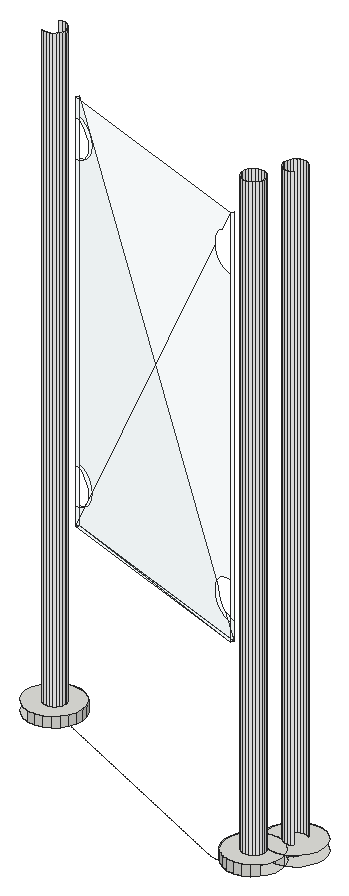
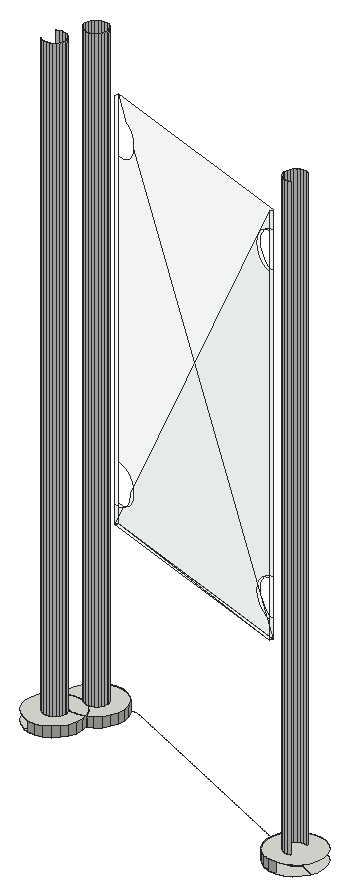
# SketchUp Ruby script. Lengths in inches.
U = 1.inch
M = Sketchup.active_model
def pt(a) = Geom::Point3d.new(a.map { |v| v * U })
def face(e, loops, mat)
  f = e.add_face(loops[0].map { |a| pt(a) })
  loops[1..].each { |l| e.add_face(l.map { |a| pt(a) }).erase! }
  f.material = f.back_material = mat if mat
  f
end
# faces: each face lists its corners as indices into pts; further lists are holes
def faces(e, pts, list, mat = nil) = list.each { |f| face(e, (f[0].is_a?(Array) ? f : [f]).map { |l| l.map { |i| pts[i] } }, mat) }
# xy, xz, yz: faces in a plane at the given z, y or x. An outline is a flat list of corners, or four numbers for a rectangle; further outlines are holes
def ring(l) = l.size == 4 ? [[l[0], l[1]], [l[2], l[1]], [l[2], l[3]], [l[0], l[3]]] : l.each_slice(2).to_a
def flat(e, list, mat, &to3) = list.each { |f| face(e, (f[0].is_a?(Array) ? f : [f]).map { |l| ring(l).map { |u, v| to3.(u, v) } }, mat) }
def xy(e, z, list, mat = nil) = flat(e, list, mat) { |x, y| [x, y, z] }
def xz(e, y, list, mat = nil) = flat(e, list, mat) { |x, z| [x, y, z] }
def yz(e, x, list, mat = nil) = flat(e, list, mat) { |y, z| [x, y, z] }
def lines(e, pts, list) = list.each { |a, b| e.add_line(pt(pts[a]), pt(pts[b])) }
# prism: a flat outline (further loops are holes) pulled along v
def prism(e, loops, v, mat = nil)
  f = face(e, loops, mat); d = Geom::Vector3d.new(v.map { |x| x * U })
  f.pushpull(f.normal.samedirection?(d) ? d.length : -d.length)
end
def box(e, o, s, mat = nil) = prism(e, [[o, [o[0] + s[0], o[1], o[2]], [o[0] + s[0], o[1] + s[1], o[2]], [o[0], o[1] + s[1], o[2]]]], [0, 0, s[2]], mat)
def at(x, y, z, deg = 0) = Geom::Transformation.translation(pt([x, y, z])) * Geom::Transformation.rotation(ORIGIN, Z_AXIS, deg.degrees)
def axes(o, x, y, z) = Geom::Transformation.new([*x, 0, *y, 0, *z, 0, *pt(o).to_a, 1])
def part(name) = M.definitions.add(name)
# library, detail: a bought-in or finely detailed component or shape, given as its bounding box
def library(name, o, s) = part(name).tap { |d| box(d.entities, o, s) }
def detail(e, o, s) = box(e.add_group.entities, o, s)
def put(e, d, t, mat = nil) = e.add_instance(d, t).tap { |i| i.material = mat if mat }
def group(e, t, mat = nil) = e.add_group.tap { |g| g.transformation = t; g.material = mat if mat }.entities
root = M.entities
M.materials.add("Glass_Safety_01").color = [204, 235, 244]
M.materials["Glass_Safety_01"].alpha = 0.1
M.materials.add("[Color_000]").color = [255, 255, 255]
xy(root,321.267,[[[843.197,534.256,843.6,534.339,843.967,534.523,844.275,534.796,844.501,535.139,844.631,535.529,844.655,535.94,844.587,536.273,844.573,536.342,844.388,536.71,844.116,537.017,843.971,537.113,843.9,537.117,843.769,537.16,843.744,537.169,843.607,537.259,843.557,537.315,843.382,537.373,842.972,537.398,842.569,537.315,842.517,537.289,842.202,537.131,841.894,536.858,841.668,536.515,841.538,536.125,841.514,535.714,841.596,535.312,841.78,534.944,841.918,534.79,842.053,534.637,842.397,534.41,842.787,534.281],[843.13,535.199,842.965,535.208,842.846,535.248,842.901,535.313,842.956,535.387,843.006,535.464,843.051,535.544,843.221,535.902,843.393,536.298,843.547,536.247,843.606,536.18,843.68,536.033,843.713,535.872,843.703,535.708,843.651,535.552,843.561,535.415,843.4375,535.305,843.291,535.232],[843.393,536.298,843.332,536.319,843.133,536.45,843.204,536.446,843.36,536.394,843.418,536.355]],[841.918,534.79,841.962,534.793,842.053,534.807,842.143,534.826,842.231,534.851,842.318,534.882,842.402,534.918,842.484,534.96,842.5625,535.007,842.638,535.059,842.71,535.116,842.778,535.177,842.842,535.243,842.846,535.248,842.809,535.26,842.672,535.351,842.563,535.474,842.489,535.621,842.456,535.782,842.466,535.946,842.518,536.102,842.608,536.239,842.731,536.349,842.878,536.422,843.039,536.455,843.133,536.45,843.204,536.446,843.36,536.394,843.418,536.355,843.769,537.16,843.744,537.169,843.607,537.259,843.557,537.315,843.498,537.382,843.424,537.529,843.391,537.69,843.401,537.854,843.453,538.01,843.543,538.148,843.666,538.257,843.813,538.331,843.974,538.364,844.139,538.354,844.27,538.31,844.645,539.173,844.317,539.282,843.907,539.306,843.504,539.223,843.137,539.039,842.829,538.766,842.603,538.423,842.473,538.033,842.449,537.623,842.517,537.289,842.202,537.131,841.894,536.858,841.668,536.515,841.538,536.125,841.514,535.714,841.596,535.312,841.78,534.944],[842.846,535.248,842.901,535.313,842.956,535.387,843.006,535.464,843.051,535.544,843.221,535.902,843.393,536.298,843.332,536.319,843.133,536.45,843.039,536.455,842.878,536.422,842.731,536.349,842.608,536.239,842.518,536.102,842.466,535.946,842.456,535.782,842.489,535.621,842.563,535.474,842.672,535.351,842.809,535.26],[[844.132,536.165,843.722,536.189,843.547,536.247,843.497,536.303,843.418,536.355,843.36,536.394,843.204,536.446,843.133,536.45,842.988,536.545,842.715,536.852,842.531,537.22,842.517,537.289,842.449,537.623,842.473,538.033,842.603,538.423,842.829,538.766,843.137,539.039,843.504,539.223,843.907,539.306,844.317,539.282,844.645,539.173,844.707,539.152,845.051,538.926,845.323,538.618,845.508,538.251,845.59,537.848,845.566,537.4375,845.436,537.047,845.21,536.704,844.902,536.431,844.587,536.273,844.535,536.247],[844.064,537.107,844.226,537.14,844.373,537.214,844.496,537.323,844.586,537.46,844.638,537.616,844.648,537.78,844.615,537.941,844.541,538.088,844.432,538.211,844.295,538.302,844.27,538.31,843.798,537.227,843.971,537.113],[843.769,537.16,843.798,537.227,843.772,537.244,843.557,537.315,843.607,537.259,843.744,537.169]],[843.769,537.16,843.744,537.169,843.607,537.259,843.557,537.315,843.772,537.244,843.798,537.227],
  [843.798,537.227,844.27,538.31,844.139,538.354,843.974,538.364,843.813,538.331,843.666,538.257,843.543,538.148,843.453,538.01,843.401,537.854,843.391,537.69,843.424,537.529,843.498,537.382,843.557,537.315,843.772,537.244],[[827.381,539.408,827.783,539.491,828.151,539.675,828.458,539.948,828.685,540.291,828.705,540.352,828.815,540.681,828.839,541.092,828.756,541.494,828.572,541.862,828.299,542.169,827.956,542.396,827.566,542.525,827.156,542.55,826.753,542.467,826.385,542.283,826.078,542.01,825.851,541.667,825.83,541.603,825.722,541.277,825.697,540.866,825.78,540.464,825.964,540.096,826.237,539.789,826.58,539.5625,826.97,539.433],[827.313,540.351,827.149,540.36,826.993,540.412,826.856,540.503,826.747,540.626,826.673,540.773,826.64,540.934,826.65,541.098,826.693,541.228,826.701,541.254,826.792,541.391,826.915,541.501,827.062,541.574,827.223,541.607,827.387,541.598,827.543,541.546,827.681,541.455,827.79,541.332,827.863,541.185,827.896,541.024,827.887,540.86,827.843,540.727,827.835,540.704,827.744,540.567,827.621,540.457,827.474,540.384]],[828.705,540.352,828.815,540.681,828.839,541.092,828.756,541.494,828.572,541.862,828.299,542.169,827.956,542.396,827.566,542.525,827.156,542.55,826.753,542.467,826.385,542.283,826.078,542.01,825.851,541.667,825.83,541.603,826.693,541.228,826.701,541.254,826.792,541.391,826.915,541.501,827.062,541.574,827.223,541.607,827.387,541.598,827.543,541.546,827.681,541.455,827.79,541.332,827.863,541.185,827.896,541.024,827.887,540.86,827.843,540.727],[827.843,540.727,827.887,540.86,827.896,541.024,827.863,541.185,827.79,541.332,827.681,541.455,827.543,541.546,827.387,541.598,827.223,541.607,827.062,541.574,826.915,541.501,826.792,541.391,826.701,541.254,826.693,541.228]])
xy(root,321.267,[[843.13,535.199,842.965,535.208,842.846,535.248,842.901,535.313,842.956,535.387,843.006,535.464,843.051,535.544,843.221,535.902,843.393,536.298,843.547,536.247,843.606,536.18,843.68,536.033,843.713,535.872,843.703,535.708,843.651,535.552,843.561,535.415,843.4375,535.305,843.291,535.232],[843.547,536.247,843.393,536.298,843.418,536.355,843.497,536.303],[843.393,536.298,843.332,536.319,843.133,536.45,843.204,536.446,843.36,536.394,843.418,536.355],[844.064,537.107,843.971,537.113,843.798,537.227,844.27,538.31,844.295,538.302,844.432,538.211,844.541,538.088,844.615,537.941,844.648,537.78,844.638,537.616,844.586,537.46,844.496,537.323,844.373,537.214,844.226,537.14],[843.971,537.113,843.798,537.227,843.769,537.16,843.9,537.117],
  [827.313,540.351,827.474,540.384,827.621,540.457,827.744,540.567,827.835,540.704,827.843,540.727,826.693,541.228,826.65,541.098,826.64,540.934,826.673,540.773,826.747,540.626,826.856,540.503,826.993,540.412,827.149,540.36]],"[Color_000]")
xy(root,321.858,[[843.197,534.256,843.6,534.339,843.967,534.523,844.275,534.796,844.501,535.139,844.631,535.529,844.655,535.94,844.587,536.273,844.535,536.247,844.132,536.165,843.722,536.189,843.332,536.319,842.988,536.545,842.715,536.852,842.531,537.22,842.517,537.289,842.202,537.131,841.894,536.858,841.668,536.515,841.538,536.125,841.514,535.714,841.596,535.312,841.78,534.944,842.053,534.637,842.397,534.41,842.787,534.281],[844.132,536.165,844.535,536.247,844.587,536.273,844.573,536.342,844.388,536.71,844.116,537.017,843.772,537.244,843.382,537.373,842.972,537.398,842.569,537.315,842.517,537.289,842.531,537.22,842.715,536.852,842.988,536.545,843.332,536.319,843.722,536.189],[844.587,536.273,844.902,536.431,845.21,536.704,845.436,537.047,845.566,537.4375,845.59,537.848,845.508,538.251,845.323,538.618,845.051,538.926,844.707,539.152,844.317,539.282,843.907,539.306,843.504,539.223,843.137,539.039,842.829,538.766,842.603,538.423,842.473,538.033,842.449,537.623,842.517,537.289,842.569,537.315,842.972,537.398,843.382,537.373,843.772,537.244,844.116,537.017,844.388,536.71,844.573,536.342],[827.381,539.408,827.783,539.491,828.151,539.675,828.458,539.948,828.685,540.291,828.815,540.681,828.839,541.092,828.756,541.494,828.572,541.862,828.299,542.169,827.956,542.396,827.566,542.525,827.156,542.55,826.753,542.467,826.385,542.283,826.078,542.01,825.851,541.667,825.722,541.277,825.697,540.866,825.78,540.464,825.964,540.096,826.237,539.789,826.58,539.5625,826.97,539.433]])
xy(root,331.897,[[841.404,536.271,829.109,540.276,829.17,540.463],[841.404,536.271,829.17,540.463,841.465,536.458],[844.039,537.551,843.862,537.638,844.044,537.562],[844.044,537.562,843.862,537.638,843.867,537.648]],"Glass_Safety_01")
p = [[842.397,534.41,321.267],[842.787,534.281,321.267],[842.787,534.281,321.858],[842.397,534.41,321.858],[843.197,534.256,321.267],[843.197,534.256,321.858],
  [843.6,534.339,321.267],[843.6,534.339,321.858],[843.967,534.523,321.267],[843.967,534.523,321.858],[842.053,534.637,321.267],[842.053,534.637,321.858],
  [844.275,534.796,321.267],[844.275,534.796,321.858],[841.78,534.944,321.267],[841.918,534.79,321.267],[841.78,534.944,321.858],[841.596,535.312,321.267],
  [841.596,535.312,321.858],[842.809,535.26,321.267],[842.846,535.248,321.267],[842.965,535.208,321.267],[842.965,535.208,357.267],[842.809,535.26,357.267],
  [843.13,535.199,321.267],[843.13,535.199,357.267],[843.291,535.232,321.267],[843.291,535.232,357.267],[843.4375,535.305,321.267],[843.4375,535.305,357.267],
  [841.514,535.714,321.267],[841.514,535.714,321.858],[842.672,535.351,321.267],[842.672,535.351,357.267],[843.561,535.415,321.267],[843.561,535.415,357.267],
  [842.563,535.474,321.267],[842.563,535.474,357.267],[843.651,535.552,321.267],[843.651,535.552,357.267],[842.489,535.621,321.267],[842.489,535.621,357.267],
  [842.456,535.782,321.267],[842.456,535.782,357.267],[843.703,535.708,321.267],[843.703,535.708,357.267],[841.538,536.125,321.267],[841.538,536.125,321.858],
  [843.713,535.872,321.267],[843.713,535.872,357.267],[842.466,535.946,321.267],[842.466,535.946,357.267],[842.518,536.102,321.267],[842.518,536.102,357.267],
  [843.68,536.033,321.267],[843.68,536.033,357.267],[843.606,536.18,321.267],[843.606,536.18,357.267],[841.668,536.515,321.267],[841.668,536.515,321.858],
  [842.608,536.239,321.267],[842.608,536.239,357.267],[842.731,536.349,321.267],[842.731,536.349,357.267],[843.332,536.319,321.267],[843.393,536.298,321.267],
  [843.547,536.247,321.267],[843.722,536.189,321.267],[843.722,536.189,321.858],[843.332,536.319,321.858],[843.497,536.303,321.267],[843.497,536.303,357.267],
  [844.132,536.165,321.267],[844.132,536.165,321.858],[844.535,536.247,321.267],[844.535,536.247,321.858],[842.878,536.422,321.267],[842.878,536.422,357.267],
  [842.988,536.545,321.267],[843.133,536.45,321.267],[842.988,536.545,321.858],[843.418,536.355,321.267],[843.36,536.394,321.267],[843.36,536.394,357.267],
  [843.039,536.455,321.267],[843.039,536.455,357.267],[843.204,536.446,321.267],[843.204,536.446,357.267],[841.894,536.858,321.267],[841.894,536.858,321.858],
  [842.715,536.852,321.267],[842.715,536.852,321.858],[844.388,536.71,321.267],[844.116,537.017,321.267],[844.116,537.017,321.858],[844.388,536.71,321.858],
  [842.202,537.131,321.267],[842.202,537.131,321.858],[842.531,537.22,321.267],[842.531,537.22,321.858],[843.971,537.113,321.267],[843.798,537.227,321.267],
  [843.772,537.244,321.267],[843.772,537.244,321.858],[842.569,537.315,321.267],[842.517,537.289,321.267],[842.517,537.289,321.858],[842.569,537.315,321.858],
  [843.744,537.169,321.267],[843.769,537.16,321.267],[843.9,537.117,321.267],[843.9,537.117,357.267],[843.744,537.169,357.267],[844.064,537.107,321.267],
  [844.064,537.107,357.267],[844.226,537.14,321.267],[844.226,537.14,357.267],[844.373,537.214,321.267],[844.373,537.214,357.267],[842.449,537.623,321.267],
  [842.449,537.623,321.858],[843.557,537.315,321.267],[843.382,537.373,321.267],[843.382,537.373,321.858],[843.607,537.259,321.267],[843.607,537.259,357.267],
  [842.972,537.398,321.267],[842.972,537.398,321.858],[843.498,537.382,321.267],[843.498,537.382,357.267],[843.424,537.529,321.267],[843.424,537.529,357.267],
  [843.391,537.69,321.267],[843.391,537.69,357.267],[842.473,538.033,321.267],[842.473,538.033,321.858],[843.401,537.854,321.267],[843.401,537.854,357.267],
  [843.453,538.01,321.267],[843.453,538.01,357.267],[842.603,538.423,321.267],[842.603,538.423,321.858],[843.543,538.148,321.267],[843.543,538.148,357.267],
  [843.666,538.257,321.267],[843.666,538.257,357.267],[844.432,538.211,321.267],[844.295,538.302,321.267],[844.295,538.302,357.267],[844.432,538.211,357.267],
  [843.813,538.331,321.267],[843.813,538.331,357.267],[843.974,538.364,321.267],[843.974,538.364,357.267],[844.27,538.31,321.267],[844.139,538.354,321.267],
  [844.139,538.354,357.267],[842.829,538.766,321.267],[842.829,538.766,321.858],[843.137,539.039,321.267],[843.137,539.039,321.858],[843.504,539.223,321.267],
  [843.504,539.223,321.858],[843.907,539.306,321.267],[843.907,539.306,321.858],[844.317,539.282,321.267],[844.317,539.282,321.858],[826.97,539.433,321.267],
  [827.381,539.408,321.267],[827.381,539.408,321.858],[826.97,539.433,321.858],[827.783,539.491,321.267],[827.783,539.491,321.858],[828.151,539.675,321.267],
  [828.151,539.675,321.858],[828.458,539.948,321.267],[828.458,539.948,321.858],[828.685,540.291,321.267],[828.685,540.291,321.858],[828.705,540.352,321.267],
  [828.815,540.681,321.267],[828.815,540.681,321.858],[826.993,540.412,321.267],[827.149,540.36,321.267],[827.149,540.36,357.267],[826.993,540.412,357.267],
  [827.313,540.351,321.267],[827.313,540.351,357.267],[827.474,540.384,321.267],[827.474,540.384,357.267],[827.621,540.457,321.267],[827.621,540.457,357.267],
  [827.744,540.567,321.267],[827.744,540.567,357.267],[827.835,540.704,321.267],[827.835,540.704,357.267],[827.843,540.727,321.267],[827.887,540.86,321.267],
  [827.887,540.86,357.267],[828.839,541.092,321.267],[828.839,541.092,321.858],[827.896,541.024,321.267],[827.896,541.024,357.267],[827.863,541.185,321.267],
  [827.863,541.185,357.267],[828.756,541.494,321.267],[828.756,541.494,321.858],[827.79,541.332,321.267],[827.79,541.332,357.267],[827.681,541.455,321.267],
  [827.681,541.455,357.267],[827.543,541.546,321.267],[827.387,541.598,321.267],[827.387,541.598,357.267],[827.543,541.546,357.267],[828.572,541.862,321.267],
  [828.572,541.862,321.858],[827.223,541.607,321.267],[827.062,541.574,321.267],[827.062,541.574,357.267],[827.223,541.607,357.267],[828.299,542.169,321.267],
  [828.299,542.169,321.858],[827.956,542.396,321.267],[827.956,542.396,321.858],[827.566,542.525,321.267],[827.566,542.525,321.858],[827.156,542.55,321.267],
  [827.156,542.55,321.858],[829.109,540.276,351.283],[829.109,540.276,335.126],[829.371,540.19,335.089],[829.615,540.111,334.983],[829.824,540.043,334.814],
  [829.985,539.991,334.594],[830.086,539.958,334.338],[830.12,539.946,334.0625],[830.086,539.958,333.787],[829.985,539.991,333.531],[829.824,540.043,333.311],
  [829.615,540.111,333.142],[829.371,540.19,333.036],[829.109,540.276,333],[829.109,540.276,331.897],[840.182,536.669,352.264],[840.172,536.672,352.346],
  [840.206,536.661,352.621],[840.307,536.628,352.877],[840.468,536.576,353.098],[840.677,536.508,353.267],[840.743,536.486,353.295],[841.404,536.271,354.511],
  [829.109,540.276,354.511],[829.109,540.276,353.409],[829.371,540.19,353.373],[829.615,540.111,353.267],[829.824,540.043,353.098],[829.985,539.991,352.877],
  [830.086,539.958,352.621],[830.12,539.946,352.346],[830.086,539.958,352.071],[829.985,539.991,351.815],[829.824,540.043,351.594],[829.615,540.111,351.425],
  [829.371,540.19,351.319],[841.404,536.271,335.126],[841.404,536.271,351.283],[841.182,536.343,351.283],[840.921,536.428,351.319],[840.677,536.508,351.425],
  [840.468,536.576,351.594],[840.307,536.628,351.815],[840.206,536.661,352.071],[841.404,536.271,331.897],[841.404,536.271,333],[841.182,536.343,333],
  [840.921,536.428,333.036],[840.677,536.508,333.142],[840.468,536.576,333.311],[840.307,536.628,333.531],[840.206,536.661,333.787],[840.172,536.672,334.0625],
  [840.206,536.661,334.338],[840.307,536.628,334.594],[840.468,536.576,334.814],[840.677,536.508,334.983],[840.921,536.428,335.089],[841.182,536.343,335.126],
  [841.465,536.458,331.897],[841.465,536.458,333],[841.465,536.458,335.126],[841.465,536.458,351.283],[841.465,536.458,353.409],[841.465,536.458,354.511],
  [841.404,536.271,353.409],[829.17,540.463,335.126],[829.17,540.463,351.283],[829.432,540.378,351.319],[829.676,540.298,351.425],[829.885,540.23,351.594],
  [830.046,540.178,351.815],[830.147,540.145,352.071],[830.181,540.134,352.346],[830.147,540.145,352.621],[830.046,540.178,352.877],[829.885,540.23,353.098],
  [829.676,540.298,353.267],[829.432,540.378,353.373],[829.17,540.463,353.409],[829.17,540.463,354.511],[840.243,536.856,334.145],[840.233,536.86,334.0625],
  [840.267,536.848,333.787],[840.368,536.815,333.531],[840.529,536.763,333.311],[840.738,536.695,333.142],[840.804,536.674,333.113],[829.17,540.463,331.897],
  [829.17,540.463,333],[829.432,540.378,333.036],[829.676,540.298,333.142],[829.885,540.23,333.311],[830.046,540.178,333.531],[830.147,540.145,333.787],
  [830.181,540.134,334.0625],[830.147,540.145,334.338],[830.046,540.178,334.594],[829.885,540.23,334.814],[829.676,540.298,334.983],[829.432,540.378,335.089],
  [840.982,536.616,333.036],[841.243,536.53,333],[843.862,537.638,331.897],[843.862,537.638,333],[843.867,537.648,333],[843.867,537.648,331.897],
  [844.039,537.551,331.897],[844.039,537.551,333],[844.039,537.552,333.078],[844.039,537.551,335.047],[844.039,537.551,335.126],[844.039,537.551,351.283],
  [844.039,537.551,351.362],[844.039,537.551,353.33],[844.039,537.551,353.409],[844.039,537.551,354.511],[843.862,537.638,354.511],[843.862,537.638,353.409],
  [843.862,537.638,353.33],[843.862,537.638,351.362],[843.862,537.638,351.283],[843.862,537.638,335.126],[843.862,537.638,335.047],[843.862,537.638,333.078],
  [844.044,537.562,331.897],[843.867,537.648,333.001],[843.867,537.648,333.078],[843.867,537.648,335.047],[843.867,537.648,335.124],[843.867,537.648,335.126],
  [843.867,537.648,351.283],[843.867,537.648,351.285],[843.867,537.648,351.362],[843.867,537.648,353.33],[843.867,537.648,353.407],[843.867,537.648,353.409],
  [843.867,537.648,354.511],[844.044,537.562,354.511],[844.044,537.561,353.409],[844.044,537.561,353.408],[844.044,537.561,353.33],[844.044,537.562,351.362],
  [844.044,537.562,351.285],[844.044,537.562,351.283],[844.044,537.562,335.126],[844.044,537.562,335.124],[844.044,537.562,335.047],[844.044,537.562,333.078],
  [844.044,537.562,333.001],[844.044,537.562,333],[840.962,535.013,321.267],[841.33,534.867,321.267],[841.417,534.839,321.267],[841.506,534.816,321.267],
  [841.596,534.8,321.267],[841.6875,534.789,321.267],[841.779,534.785,321.267],[841.871,534.786,321.267]]
faces(root,p,[[0,1,2,3],[1,4,5,2],[4,6,7,5],[6,8,9,7],[10,0,3,11],[8,12,13,9],[14,15,10,11,16],[17,14,16,18],
  [30,17,18,31],[46,30,31,47],[58,46,47,59],[64,65,66,67,68,69],[67,72,73,68],[72,74,75,73],[78,79,64,69,80],[88,58,59,89],
  [90,78,80,91],[92,93,94,95],[96,88,89,97],[98,90,91,99],[93,100,101,102,103,94],[104,105,96,97,106,107],[119,105,98,99,106,120],[102,121,122,123,103],
  [126,104,107,127],[122,126,127,123],[134,119,120,135],[140,134,135,141],[157,140,141,158],[159,157,158,160],[161,159,160,162],[163,161,162,164],
  [165,163,164,166],[167,168,169,170],[168,171,172,169],[171,173,174,172],[173,175,176,174],[175,177,178,176],[177,179,180,181,178],[180,199,200,181],
  [199,205,206,200],[205,215,216,206],[215,221,222,216],[221,223,224,222],[223,225,226,224],[225,227,228,226]])
faces(root,p,[[19,20,21,22,23],[21,24,25,22],[24,26,27,25],[26,28,29,27],[32,19,23,33],[28,34,35,29],[36,32,33,37],[34,38,39,35],
  [40,36,37,41],[42,40,41,43],[38,44,45,39],[44,48,49,45],[50,42,43,51],[52,50,51,53],[48,54,55,49],[54,56,57,55],
  [60,52,53,61],[62,60,61,63],[56,66,70,71,57],[76,62,63,77],[70,81,82,83,71],[84,76,77,85],[86,79,84,85,87],[82,86,87,83],
  [108,109,110,111,112],[110,100,113,114,111],[113,115,116,114],[115,117,118,116],[124,108,112,125],[128,121,124,125,129],[130,128,129,131],[132,130,131,133],
  [136,132,133,137],[138,136,137,139],[142,138,139,143],[144,142,143,145],[146,147,148,149],[150,144,145,151],[152,150,151,153],[147,154,155,156,148],
  [155,152,153,156],[182,183,184,185],[183,186,187,184],[186,188,189,187],[188,190,191,189],[190,192,193,191],[192,194,195,193],[194,196,197,198,195],
  [197,201,202,198],[201,203,204,202],[203,207,208,204],[207,209,210,208],[211,212,213,214],[209,211,214,210],[217,218,219,220],[212,217,220,213]],"[Color_000]")
faces(root,p,[[229,230,231,232,233,234,235,236,237,238,239,240,241,242,243,244,245,246,247,248,249,250,251,252,253,254,255,256,257,258,259,260,261,262,263,264],[265,266,267,268,269,270,271,272,244,243,273,274,275,276,277,278,279,280,281,282,283,284,285,286,287],[273,288,289,290,291,292,293,251,294,266,265,274],[295,296,297,298,299,300,301,302,303,304,305,306,307,308,309,310,311,312,313,314,315,316,288,317,318,319,320,321,322,323,324,325,326,327,328,329],[288,316,330,331,289],[332,333,334,335],[332,336,337,338,339,340,341,342,343,344,345,346,347,348,349,350,351,352,353,333],[354,335,334,355,356,357,358,359,360,361,362,363,364,365,366,367,368,369,370,371,372,373,374,375,376,377,378,379],
  [354,379,337,336],[317,243,242,230,229,253,252,309,308,296,295,318]],"Glass_Safety_01")
lines(root,p,[[380,381],[381,382],[382,383],[383,384],[384,385],[385,386],[386,387],[387,15],[179,380]])
